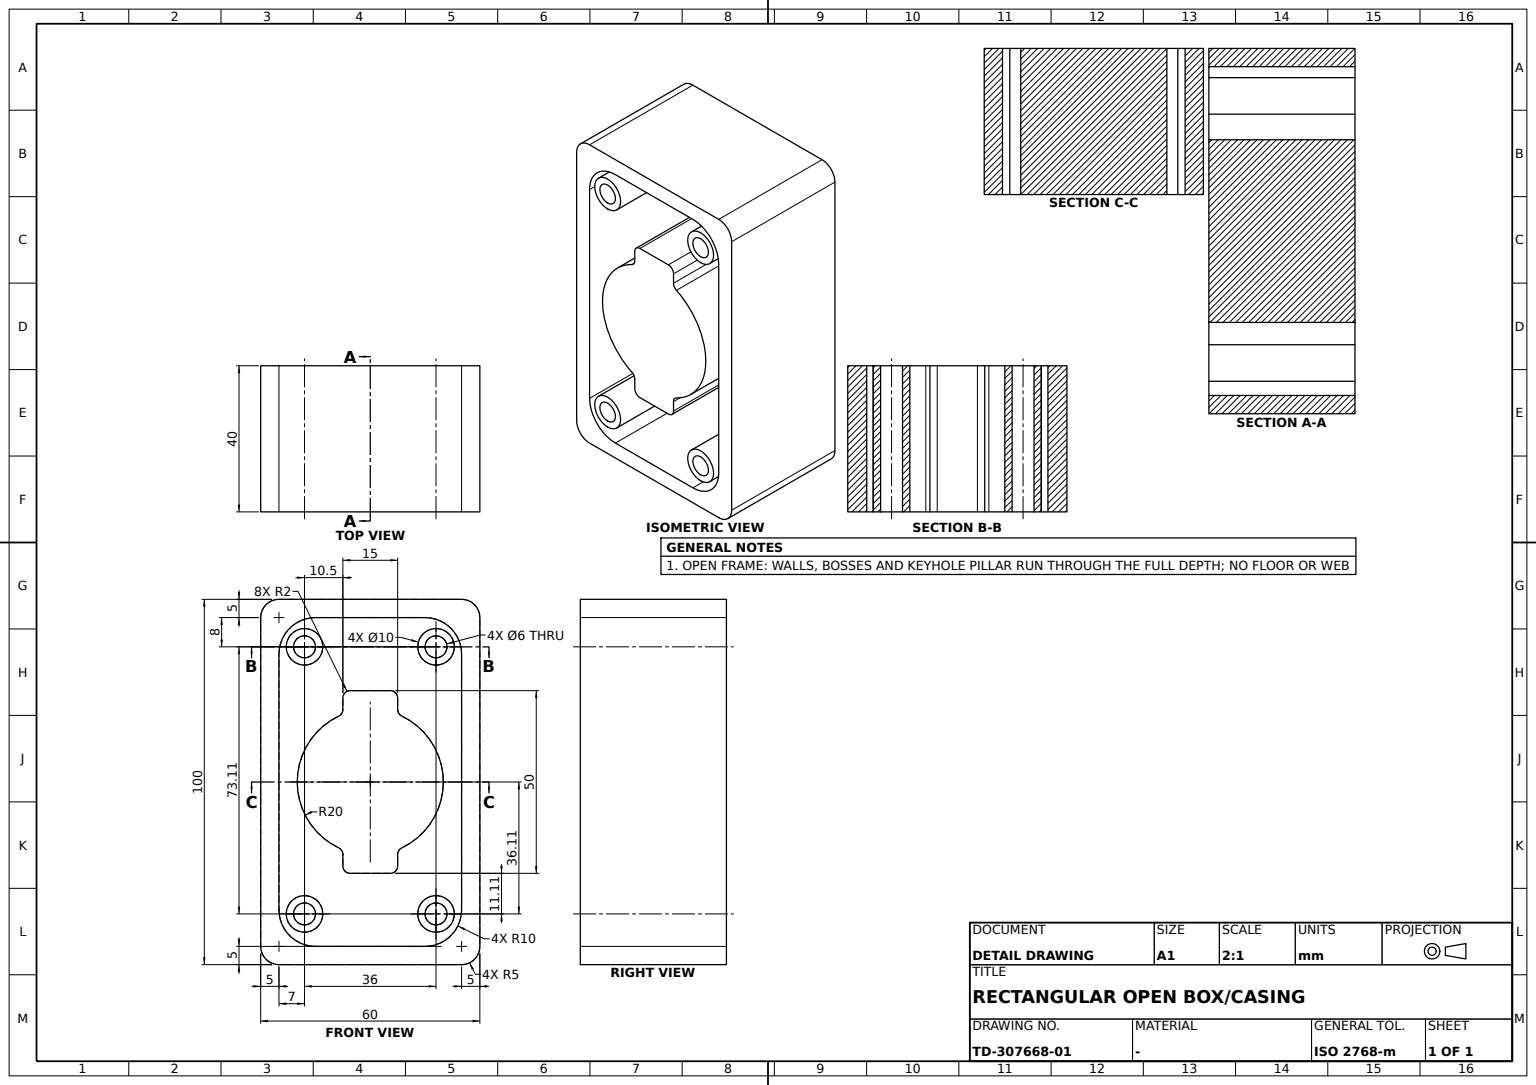
ISO-10303-21;
HEADER;
FILE_DESCRIPTION((''),'2;1');
FILE_NAME('','',(''),(''),'','','');
FILE_SCHEMA(('AUTOMOTIVE_DESIGN'));
ENDSEC;
DATA;
#1=APPLICATION_CONTEXT('');
#2=PRODUCT_CONTEXT('',#1,'mechanical');
#3=PRODUCT('','','',(#2));
#4=PRODUCT_DEFINITION_FORMATION('','',#3);
#5=PRODUCT_DEFINITION_CONTEXT('',#1,'design');
#6=PRODUCT_DEFINITION('','',#4,#5);
#7=PRODUCT_DEFINITION_SHAPE('','',#6);
#8=(LENGTH_UNIT()NAMED_UNIT(*)SI_UNIT(.MILLI.,.METRE.));
#9=(NAMED_UNIT(*)PLANE_ANGLE_UNIT()SI_UNIT($,.RADIAN.));
#10=(NAMED_UNIT(*)SI_UNIT($,.STERADIAN.)SOLID_ANGLE_UNIT());
#11=UNCERTAINTY_MEASURE_WITH_UNIT(LENGTH_MEASURE(0.005),#8,'distance_accuracy_value','');
#12=(GEOMETRIC_REPRESENTATION_CONTEXT(3)GLOBAL_UNCERTAINTY_ASSIGNED_CONTEXT((#11))GLOBAL_UNIT_ASSIGNED_CONTEXT((#8,#9,#10))REPRESENTATION_CONTEXT('',''));
#13=CARTESIAN_POINT('',(20.,-18.,-41.111401));
#14=VERTEX_POINT('',#13);
#15=CARTESIAN_POINT('',(20.,-18.,-36.111401));
#16=DIRECTION('',(1.,0.,0.));
#17=DIRECTION('',(0.,0.,-1.));
#18=AXIS2_PLACEMENT_3D('',#15,#16,#17);
#19=CIRCLE('',#18,5.);
#20=EDGE_CURVE('',#14,#14,#19,.T.);
#21=ORIENTED_EDGE('',*,*,#20,.T.);
#22=EDGE_LOOP('',(#21));
#23=FACE_BOUND('',#22,.T.);
#24=CARTESIAN_POINT('',(20.,-18.,-39.111401));
#25=VERTEX_POINT('',#24);
#26=CIRCLE('',#18,3.);
#27=EDGE_CURVE('',#25,#25,#26,.T.);
#28=ORIENTED_EDGE('',*,*,#27,.F.);
#29=EDGE_LOOP('',(#28));
#30=FACE_BOUND('',#29,.T.);
#31=CARTESIAN_POINT('',(20.,0.,0.));
#32=DIRECTION('',(0.,1.,0.));
#33=AXIS2_PLACEMENT_3D('',#31,#16,#32);
#34=PLANE('',#33);
#35=ADVANCED_FACE('',(#23,#30),#34,.T.);
#36=ORIENTED_EDGE('',*,*,#20,.F.);
#37=EDGE_LOOP('',(#36));
#38=FACE_BOUND('',#37,.T.);
#39=CARTESIAN_POINT('',(-20.,-18.,-41.111401));
#40=VERTEX_POINT('',#39);
#41=CARTESIAN_POINT('',(-20.,-18.,-36.111401));
#42=AXIS2_PLACEMENT_3D('',#41,#16,#17);
#43=CIRCLE('',#42,5.);
#44=EDGE_CURVE('',#40,#40,#43,.T.);
#45=ORIENTED_EDGE('',*,*,#44,.T.);
#46=EDGE_LOOP('',(#45));
#47=FACE_BOUND('',#46,.T.);
#48=CARTESIAN_POINT('',(0.,-18.,-36.111401));
#49=AXIS2_PLACEMENT_3D('',#48,#16,#32);
#50=CYLINDRICAL_SURFACE('',#49,5.);
#51=ADVANCED_FACE('',(#38,#47),#50,.T.);
#52=ORIENTED_EDGE('',*,*,#44,.F.);
#53=EDGE_LOOP('',(#52));
#54=FACE_BOUND('',#53,.T.);
#55=CARTESIAN_POINT('',(-20.,-18.,-39.111401));
#56=VERTEX_POINT('',#55);
#57=CIRCLE('',#42,3.);
#58=EDGE_CURVE('',#56,#56,#57,.T.);
#59=ORIENTED_EDGE('',*,*,#58,.T.);
#60=EDGE_LOOP('',(#59));
#61=FACE_BOUND('',#60,.T.);
#62=CARTESIAN_POINT('',(-20.,0.,0.));
#63=AXIS2_PLACEMENT_3D('',#62,#16,#32);
#64=PLANE('',#63);
#65=ADVANCED_FACE('',(#54,#61),#64,.F.);
#66=ORIENTED_EDGE('',*,*,#27,.T.);
#67=EDGE_LOOP('',(#66));
#68=FACE_BOUND('',#67,.T.);
#69=ORIENTED_EDGE('',*,*,#58,.F.);
#70=EDGE_LOOP('',(#69));
#71=FACE_BOUND('',#70,.T.);
#72=CYLINDRICAL_SURFACE('',#49,3.);
#73=ADVANCED_FACE('',(#68,#71),#72,.F.);
#74=CLOSED_SHELL('',(#35,#51,#65,#73));
#75=MANIFOLD_SOLID_BREP('',#74);
#76=CARTESIAN_POINT('',(-20.,30.,45.));
#77=VERTEX_POINT('',#76);
#78=CARTESIAN_POINT('',(20.,30.,45.));
#79=VERTEX_POINT('',#78);
#80=CARTESIAN_POINT('',(0.,30.,45.));
#81=VECTOR('',#16,1000.);
#82=LINE('',#80,#81);
#83=EDGE_CURVE('',#77,#79,#82,.T.);
#84=ORIENTED_EDGE('',*,*,#83,.T.);
#85=CARTESIAN_POINT('',(20.,30.,-45.));
#86=VERTEX_POINT('',#85);
#87=CARTESIAN_POINT('',(20.,30.,0.));
#88=DIRECTION('',(0.,0.,1.));
#89=VECTOR('',#88,1000.);
#90=LINE('',#87,#89);
#91=EDGE_CURVE('',#86,#79,#90,.T.);
#92=ORIENTED_EDGE('',*,*,#91,.F.);
#93=CARTESIAN_POINT('',(-20.,30.,-45.));
#94=VERTEX_POINT('',#93);
#95=CARTESIAN_POINT('',(0.,30.,-45.));
#96=LINE('',#95,#81);
#97=EDGE_CURVE('',#94,#86,#96,.T.);
#98=ORIENTED_EDGE('',*,*,#97,.F.);
#99=CARTESIAN_POINT('',(-20.,30.,0.));
#100=LINE('',#99,#89);
#101=EDGE_CURVE('',#94,#77,#100,.T.);
#102=ORIENTED_EDGE('',*,*,#101,.T.);
#103=EDGE_LOOP('',(#84,#92,#98,#102));
#104=FACE_BOUND('',#103,.T.);
#105=CARTESIAN_POINT('',(0.,30.,-50.));
#106=AXIS2_PLACEMENT_3D('',#105,#32,#88);
#107=PLANE('',#106);
#108=ADVANCED_FACE('',(#104),#107,.T.);
#109=CARTESIAN_POINT('',(-20.,25.,35.));
#110=VERTEX_POINT('',#109);
#111=CARTESIAN_POINT('',(20.,25.,35.));
#112=VERTEX_POINT('',#111);
#113=CARTESIAN_POINT('',(0.,25.,35.));
#114=LINE('',#113,#81);
#115=EDGE_CURVE('',#110,#112,#114,.T.);
#116=ORIENTED_EDGE('',*,*,#115,.F.);
#117=CARTESIAN_POINT('',(-20.,25.,-35.));
#118=VERTEX_POINT('',#117);
#119=CARTESIAN_POINT('',(-20.,25.,0.));
#120=LINE('',#119,#89);
#121=EDGE_CURVE('',#118,#110,#120,.T.);
#122=ORIENTED_EDGE('',*,*,#121,.F.);
#123=CARTESIAN_POINT('',(20.,25.,-35.));
#124=VERTEX_POINT('',#123);
#125=CARTESIAN_POINT('',(0.,25.,-35.));
#126=LINE('',#125,#81);
#127=EDGE_CURVE('',#118,#124,#126,.T.);
#128=ORIENTED_EDGE('',*,*,#127,.T.);
#129=CARTESIAN_POINT('',(20.,25.,0.));
#130=LINE('',#129,#89);
#131=EDGE_CURVE('',#124,#112,#130,.T.);
#132=ORIENTED_EDGE('',*,*,#131,.T.);
#133=EDGE_LOOP('',(#116,#122,#128,#132));
#134=FACE_BOUND('',#133,.T.);
#135=CARTESIAN_POINT('',(0.,25.,-45.));
#136=AXIS2_PLACEMENT_3D('',#135,#32,#88);
#137=PLANE('',#136);
#138=ADVANCED_FACE('',(#134),#137,.F.);
#139=CARTESIAN_POINT('',(-20.,-30.,-45.));
#140=VERTEX_POINT('',#139);
#141=CARTESIAN_POINT('',(20.,-30.,-45.));
#142=VERTEX_POINT('',#141);
#143=CARTESIAN_POINT('',(0.,-30.,-45.));
#144=LINE('',#143,#81);
#145=EDGE_CURVE('',#140,#142,#144,.T.);
#146=ORIENTED_EDGE('',*,*,#145,.F.);
#147=CARTESIAN_POINT('',(-20.,-25.,-50.));
#148=VERTEX_POINT('',#147);
#149=CARTESIAN_POINT('',(-20.,-25.,-45.));
#150=AXIS2_PLACEMENT_3D('',#149,#16,#17);
#151=CIRCLE('',#150,5.);
#152=EDGE_CURVE('',#140,#148,#151,.T.);
#153=ORIENTED_EDGE('',*,*,#152,.T.);
#154=CARTESIAN_POINT('',(20.,-25.,-50.));
#155=VERTEX_POINT('',#154);
#156=CARTESIAN_POINT('',(0.,-25.,-50.));
#157=LINE('',#156,#81);
#158=EDGE_CURVE('',#148,#155,#157,.T.);
#159=ORIENTED_EDGE('',*,*,#158,.T.);
#160=CARTESIAN_POINT('',(20.,-25.,-45.));
#161=AXIS2_PLACEMENT_3D('',#160,#16,#17);
#162=CIRCLE('',#161,5.);
#163=EDGE_CURVE('',#142,#155,#162,.T.);
#164=ORIENTED_EDGE('',*,*,#163,.F.);
#165=EDGE_LOOP('',(#146,#153,#159,#164));
#166=FACE_BOUND('',#165,.T.);
#167=CARTESIAN_POINT('',(0.,-25.,-45.));
#168=AXIS2_PLACEMENT_3D('',#167,#16,#17);
#169=CYLINDRICAL_SURFACE('',#168,5.);
#170=ADVANCED_FACE('',(#166),#169,.T.);
#171=CARTESIAN_POINT('',(20.,15.,-45.));
#172=VERTEX_POINT('',#171);
#173=CARTESIAN_POINT('',(20.,15.,-35.));
#174=AXIS2_PLACEMENT_3D('',#173,#16,#17);
#175=CIRCLE('',#174,10.);
#176=EDGE_CURVE('',#172,#124,#175,.T.);
#177=ORIENTED_EDGE('',*,*,#176,.T.);
#178=ORIENTED_EDGE('',*,*,#127,.F.);
#179=CARTESIAN_POINT('',(-20.,15.,-45.));
#180=VERTEX_POINT('',#179);
#181=CARTESIAN_POINT('',(-20.,15.,-35.));
#182=AXIS2_PLACEMENT_3D('',#181,#16,#17);
#183=CIRCLE('',#182,10.);
#184=EDGE_CURVE('',#180,#118,#183,.T.);
#185=ORIENTED_EDGE('',*,*,#184,.F.);
#186=CARTESIAN_POINT('',(0.,15.,-45.));
#187=LINE('',#186,#81);
#188=EDGE_CURVE('',#180,#172,#187,.T.);
#189=ORIENTED_EDGE('',*,*,#188,.T.);
#190=EDGE_LOOP('',(#177,#178,#185,#189));
#191=FACE_BOUND('',#190,.T.);
#192=CARTESIAN_POINT('',(0.,15.,-35.));
#193=AXIS2_PLACEMENT_3D('',#192,#16,#17);
#194=CYLINDRICAL_SURFACE('',#193,10.);
#195=ADVANCED_FACE('',(#191),#194,.F.);
#196=CARTESIAN_POINT('',(20.,25.,-50.));
#197=VERTEX_POINT('',#196);
#198=CARTESIAN_POINT('',(20.,0.,-50.));
#199=DIRECTION('',(0.,-1.,0.));
#200=VECTOR('',#199,1000.);
#201=LINE('',#198,#200);
#202=EDGE_CURVE('',#197,#155,#201,.T.);
#203=ORIENTED_EDGE('',*,*,#202,.F.);
#204=CARTESIAN_POINT('',(20.,25.,-45.));
#205=AXIS2_PLACEMENT_3D('',#204,#16,#17);
#206=CIRCLE('',#205,5.);
#207=EDGE_CURVE('',#197,#86,#206,.T.);
#208=ORIENTED_EDGE('',*,*,#207,.T.);
#209=ORIENTED_EDGE('',*,*,#91,.T.);
#210=CARTESIAN_POINT('',(20.,25.,50.));
#211=VERTEX_POINT('',#210);
#212=CARTESIAN_POINT('',(20.,25.,45.));
#213=AXIS2_PLACEMENT_3D('',#212,#16,#17);
#214=CIRCLE('',#213,5.);
#215=EDGE_CURVE('',#79,#211,#214,.T.);
#216=ORIENTED_EDGE('',*,*,#215,.T.);
#217=CARTESIAN_POINT('',(20.,-25.,50.));
#218=VERTEX_POINT('',#217);
#219=CARTESIAN_POINT('',(20.,0.,50.));
#220=VECTOR('',#32,1000.);
#221=LINE('',#219,#220);
#222=EDGE_CURVE('',#218,#211,#221,.T.);
#223=ORIENTED_EDGE('',*,*,#222,.F.);
#224=CARTESIAN_POINT('',(20.,-30.,45.));
#225=VERTEX_POINT('',#224);
#226=CARTESIAN_POINT('',(20.,-25.,45.));
#227=AXIS2_PLACEMENT_3D('',#226,#16,#17);
#228=CIRCLE('',#227,5.);
#229=EDGE_CURVE('',#218,#225,#228,.T.);
#230=ORIENTED_EDGE('',*,*,#229,.T.);
#231=CARTESIAN_POINT('',(20.,-30.,0.));
#232=VECTOR('',#17,1000.);
#233=LINE('',#231,#232);
#234=EDGE_CURVE('',#225,#142,#233,.T.);
#235=ORIENTED_EDGE('',*,*,#234,.T.);
#236=ORIENTED_EDGE('',*,*,#163,.T.);
#237=EDGE_LOOP('',(#203,#208,#209,#216,#223,#230,#235,#236));
#238=FACE_BOUND('',#237,.T.);
#239=CARTESIAN_POINT('',(20.,-15.,45.));
#240=VERTEX_POINT('',#239);
#241=CARTESIAN_POINT('',(20.,-25.,35.));
#242=VERTEX_POINT('',#241);
#243=CARTESIAN_POINT('',(20.,-15.,35.));
#244=AXIS2_PLACEMENT_3D('',#243,#16,#17);
#245=CIRCLE('',#244,10.);
#246=EDGE_CURVE('',#240,#242,#245,.T.);
#247=ORIENTED_EDGE('',*,*,#246,.F.);
#248=CARTESIAN_POINT('',(20.,15.,45.));
#249=VERTEX_POINT('',#248);
#250=CARTESIAN_POINT('',(20.,0.,45.));
#251=LINE('',#250,#220);
#252=EDGE_CURVE('',#240,#249,#251,.T.);
#253=ORIENTED_EDGE('',*,*,#252,.T.);
#254=CARTESIAN_POINT('',(20.,15.,35.));
#255=AXIS2_PLACEMENT_3D('',#254,#16,#17);
#256=CIRCLE('',#255,10.);
#257=EDGE_CURVE('',#112,#249,#256,.T.);
#258=ORIENTED_EDGE('',*,*,#257,.F.);
#259=ORIENTED_EDGE('',*,*,#131,.F.);
#260=ORIENTED_EDGE('',*,*,#176,.F.);
#261=CARTESIAN_POINT('',(20.,-15.,-45.));
#262=VERTEX_POINT('',#261);
#263=CARTESIAN_POINT('',(20.,0.,-45.));
#264=LINE('',#263,#200);
#265=EDGE_CURVE('',#172,#262,#264,.T.);
#266=ORIENTED_EDGE('',*,*,#265,.T.);
#267=CARTESIAN_POINT('',(20.,-25.,-35.));
#268=VERTEX_POINT('',#267);
#269=CARTESIAN_POINT('',(20.,-15.,-35.));
#270=AXIS2_PLACEMENT_3D('',#269,#16,#17);
#271=CIRCLE('',#270,10.);
#272=EDGE_CURVE('',#268,#262,#271,.T.);
#273=ORIENTED_EDGE('',*,*,#272,.F.);
#274=CARTESIAN_POINT('',(20.,-25.,0.));
#275=LINE('',#274,#232);
#276=EDGE_CURVE('',#242,#268,#275,.T.);
#277=ORIENTED_EDGE('',*,*,#276,.F.);
#278=EDGE_LOOP('',(#247,#253,#258,#259,#260,#266,#273,#277));
#279=FACE_BOUND('',#278,.T.);
#280=ADVANCED_FACE('',(#238,#279),#34,.T.);
#281=ORIENTED_EDGE('',*,*,#252,.F.);
#282=CARTESIAN_POINT('',(-20.,-15.,45.));
#283=VERTEX_POINT('',#282);
#284=CARTESIAN_POINT('',(0.,-15.,45.));
#285=LINE('',#284,#81);
#286=EDGE_CURVE('',#283,#240,#285,.T.);
#287=ORIENTED_EDGE('',*,*,#286,.F.);
#288=CARTESIAN_POINT('',(-20.,15.,45.));
#289=VERTEX_POINT('',#288);
#290=CARTESIAN_POINT('',(-20.,0.,45.));
#291=LINE('',#290,#220);
#292=EDGE_CURVE('',#283,#289,#291,.T.);
#293=ORIENTED_EDGE('',*,*,#292,.T.);
#294=CARTESIAN_POINT('',(0.,15.,45.));
#295=LINE('',#294,#81);
#296=EDGE_CURVE('',#289,#249,#295,.T.);
#297=ORIENTED_EDGE('',*,*,#296,.T.);
#298=EDGE_LOOP('',(#281,#287,#293,#297));
#299=FACE_BOUND('',#298,.T.);
#300=CARTESIAN_POINT('',(0.,-25.,45.));
#301=AXIS2_PLACEMENT_3D('',#300,#17,#32);
#302=PLANE('',#301);
#303=ADVANCED_FACE('',(#299),#302,.T.);
#304=CARTESIAN_POINT('',(-20.,-25.,50.));
#305=VERTEX_POINT('',#304);
#306=CARTESIAN_POINT('',(-20.,-30.,45.));
#307=VERTEX_POINT('',#306);
#308=CARTESIAN_POINT('',(-20.,-25.,45.));
#309=AXIS2_PLACEMENT_3D('',#308,#16,#17);
#310=CIRCLE('',#309,5.);
#311=EDGE_CURVE('',#305,#307,#310,.T.);
#312=ORIENTED_EDGE('',*,*,#311,.T.);
#313=CARTESIAN_POINT('',(0.,-30.,45.));
#314=LINE('',#313,#81);
#315=EDGE_CURVE('',#307,#225,#314,.T.);
#316=ORIENTED_EDGE('',*,*,#315,.T.);
#317=ORIENTED_EDGE('',*,*,#229,.F.);
#318=CARTESIAN_POINT('',(0.,-25.,50.));
#319=LINE('',#318,#81);
#320=EDGE_CURVE('',#305,#218,#319,.T.);
#321=ORIENTED_EDGE('',*,*,#320,.F.);
#322=EDGE_LOOP('',(#312,#316,#317,#321));
#323=FACE_BOUND('',#322,.T.);
#324=AXIS2_PLACEMENT_3D('',#300,#16,#199);
#325=CYLINDRICAL_SURFACE('',#324,5.);
#326=ADVANCED_FACE('',(#323),#325,.T.);
#327=CARTESIAN_POINT('',(-20.,-25.,35.));
#328=VERTEX_POINT('',#327);
#329=CARTESIAN_POINT('',(0.,-25.,35.));
#330=LINE('',#329,#81);
#331=EDGE_CURVE('',#328,#242,#330,.T.);
#332=ORIENTED_EDGE('',*,*,#331,.T.);
#333=ORIENTED_EDGE('',*,*,#276,.T.);
#334=CARTESIAN_POINT('',(-20.,-25.,-35.));
#335=VERTEX_POINT('',#334);
#336=CARTESIAN_POINT('',(0.,-25.,-35.));
#337=LINE('',#336,#81);
#338=EDGE_CURVE('',#335,#268,#337,.T.);
#339=ORIENTED_EDGE('',*,*,#338,.F.);
#340=CARTESIAN_POINT('',(-20.,-25.,0.));
#341=LINE('',#340,#232);
#342=EDGE_CURVE('',#328,#335,#341,.T.);
#343=ORIENTED_EDGE('',*,*,#342,.F.);
#344=EDGE_LOOP('',(#332,#333,#339,#343));
#345=FACE_BOUND('',#344,.T.);
#346=AXIS2_PLACEMENT_3D('',#300,#199,#17);
#347=PLANE('',#346);
#348=ADVANCED_FACE('',(#345),#347,.F.);
#349=CARTESIAN_POINT('',(-20.,-15.,-45.));
#350=VERTEX_POINT('',#349);
#351=CARTESIAN_POINT('',(0.,-15.,-45.));
#352=LINE('',#351,#81);
#353=EDGE_CURVE('',#350,#262,#352,.T.);
#354=ORIENTED_EDGE('',*,*,#353,.F.);
#355=CARTESIAN_POINT('',(-20.,-15.,-35.));
#356=AXIS2_PLACEMENT_3D('',#355,#16,#17);
#357=CIRCLE('',#356,10.);
#358=EDGE_CURVE('',#335,#350,#357,.T.);
#359=ORIENTED_EDGE('',*,*,#358,.F.);
#360=ORIENTED_EDGE('',*,*,#338,.T.);
#361=ORIENTED_EDGE('',*,*,#272,.T.);
#362=EDGE_LOOP('',(#354,#359,#360,#361));
#363=FACE_BOUND('',#362,.T.);
#364=CARTESIAN_POINT('',(0.,-15.,-35.));
#365=AXIS2_PLACEMENT_3D('',#364,#16,#199);
#366=CYLINDRICAL_SURFACE('',#365,10.);
#367=ADVANCED_FACE('',(#363),#366,.F.);
#368=ORIENTED_EDGE('',*,*,#234,.F.);
#369=ORIENTED_EDGE('',*,*,#315,.F.);
#370=CARTESIAN_POINT('',(-20.,-30.,0.));
#371=LINE('',#370,#232);
#372=EDGE_CURVE('',#307,#140,#371,.T.);
#373=ORIENTED_EDGE('',*,*,#372,.T.);
#374=ORIENTED_EDGE('',*,*,#145,.T.);
#375=EDGE_LOOP('',(#368,#369,#373,#374));
#376=FACE_BOUND('',#375,.T.);
#377=CARTESIAN_POINT('',(0.,-30.,50.));
#378=AXIS2_PLACEMENT_3D('',#377,#199,#17);
#379=PLANE('',#378);
#380=ADVANCED_FACE('',(#376),#379,.T.);
#381=ORIENTED_EDGE('',*,*,#331,.F.);
#382=CARTESIAN_POINT('',(-20.,-15.,35.));
#383=AXIS2_PLACEMENT_3D('',#382,#16,#17);
#384=CIRCLE('',#383,10.);
#385=EDGE_CURVE('',#283,#328,#384,.T.);
#386=ORIENTED_EDGE('',*,*,#385,.F.);
#387=ORIENTED_EDGE('',*,*,#286,.T.);
#388=ORIENTED_EDGE('',*,*,#246,.T.);
#389=EDGE_LOOP('',(#381,#386,#387,#388));
#390=FACE_BOUND('',#389,.T.);
#391=CARTESIAN_POINT('',(0.,-15.,35.));
#392=AXIS2_PLACEMENT_3D('',#391,#16,#88);
#393=CYLINDRICAL_SURFACE('',#392,10.);
#394=ADVANCED_FACE('',(#390),#393,.F.);
#395=ORIENTED_EDGE('',*,*,#353,.T.);
#396=ORIENTED_EDGE('',*,*,#265,.F.);
#397=ORIENTED_EDGE('',*,*,#188,.F.);
#398=CARTESIAN_POINT('',(-20.,0.,-45.));
#399=LINE('',#398,#200);
#400=EDGE_CURVE('',#180,#350,#399,.T.);
#401=ORIENTED_EDGE('',*,*,#400,.T.);
#402=EDGE_LOOP('',(#395,#396,#397,#401));
#403=FACE_BOUND('',#402,.T.);
#404=AXIS2_PLACEMENT_3D('',#135,#88,#199);
#405=PLANE('',#404);
#406=ADVANCED_FACE('',(#403),#405,.T.);
#407=CARTESIAN_POINT('',(-20.,25.,50.));
#408=VERTEX_POINT('',#407);
#409=CARTESIAN_POINT('',(0.,25.,50.));
#410=LINE('',#409,#81);
#411=EDGE_CURVE('',#408,#211,#410,.T.);
#412=ORIENTED_EDGE('',*,*,#411,.F.);
#413=CARTESIAN_POINT('',(-20.,0.,50.));
#414=LINE('',#413,#220);
#415=EDGE_CURVE('',#305,#408,#414,.T.);
#416=ORIENTED_EDGE('',*,*,#415,.F.);
#417=ORIENTED_EDGE('',*,*,#320,.T.);
#418=ORIENTED_EDGE('',*,*,#222,.T.);
#419=EDGE_LOOP('',(#412,#416,#417,#418));
#420=FACE_BOUND('',#419,.T.);
#421=AXIS2_PLACEMENT_3D('',#377,#17,#32);
#422=PLANE('',#421);
#423=ADVANCED_FACE('',(#420),#422,.F.);
#424=ORIENTED_EDGE('',*,*,#202,.T.);
#425=ORIENTED_EDGE('',*,*,#158,.F.);
#426=CARTESIAN_POINT('',(-20.,25.,-50.));
#427=VERTEX_POINT('',#426);
#428=CARTESIAN_POINT('',(-20.,0.,-50.));
#429=LINE('',#428,#200);
#430=EDGE_CURVE('',#427,#148,#429,.T.);
#431=ORIENTED_EDGE('',*,*,#430,.F.);
#432=CARTESIAN_POINT('',(0.,25.,-50.));
#433=LINE('',#432,#81);
#434=EDGE_CURVE('',#427,#197,#433,.T.);
#435=ORIENTED_EDGE('',*,*,#434,.T.);
#436=EDGE_LOOP('',(#424,#425,#431,#435));
#437=FACE_BOUND('',#436,.T.);
#438=AXIS2_PLACEMENT_3D('',#105,#88,#199);
#439=PLANE('',#438);
#440=ADVANCED_FACE('',(#437),#439,.F.);
#441=ORIENTED_EDGE('',*,*,#415,.T.);
#442=CARTESIAN_POINT('',(-20.,25.,45.));
#443=AXIS2_PLACEMENT_3D('',#442,#16,#17);
#444=CIRCLE('',#443,5.);
#445=EDGE_CURVE('',#77,#408,#444,.T.);
#446=ORIENTED_EDGE('',*,*,#445,.F.);
#447=ORIENTED_EDGE('',*,*,#101,.F.);
#448=CARTESIAN_POINT('',(-20.,25.,-45.));
#449=AXIS2_PLACEMENT_3D('',#448,#16,#17);
#450=CIRCLE('',#449,5.);
#451=EDGE_CURVE('',#427,#94,#450,.T.);
#452=ORIENTED_EDGE('',*,*,#451,.F.);
#453=ORIENTED_EDGE('',*,*,#430,.T.);
#454=ORIENTED_EDGE('',*,*,#152,.F.);
#455=ORIENTED_EDGE('',*,*,#372,.F.);
#456=ORIENTED_EDGE('',*,*,#311,.F.);
#457=EDGE_LOOP('',(#441,#446,#447,#452,#453,#454,#455,#456));
#458=FACE_BOUND('',#457,.T.);
#459=ORIENTED_EDGE('',*,*,#342,.T.);
#460=ORIENTED_EDGE('',*,*,#358,.T.);
#461=ORIENTED_EDGE('',*,*,#400,.F.);
#462=ORIENTED_EDGE('',*,*,#184,.T.);
#463=ORIENTED_EDGE('',*,*,#121,.T.);
#464=CARTESIAN_POINT('',(-20.,15.,35.));
#465=AXIS2_PLACEMENT_3D('',#464,#16,#17);
#466=CIRCLE('',#465,10.);
#467=EDGE_CURVE('',#110,#289,#466,.T.);
#468=ORIENTED_EDGE('',*,*,#467,.T.);
#469=ORIENTED_EDGE('',*,*,#292,.F.);
#470=ORIENTED_EDGE('',*,*,#385,.T.);
#471=EDGE_LOOP('',(#459,#460,#461,#462,#463,#468,#469,#470));
#472=FACE_BOUND('',#471,.T.);
#473=ADVANCED_FACE('',(#458,#472),#64,.F.);
#474=ORIENTED_EDGE('',*,*,#411,.T.);
#475=ORIENTED_EDGE('',*,*,#215,.F.);
#476=ORIENTED_EDGE('',*,*,#83,.F.);
#477=ORIENTED_EDGE('',*,*,#445,.T.);
#478=EDGE_LOOP('',(#474,#475,#476,#477));
#479=FACE_BOUND('',#478,.T.);
#480=CARTESIAN_POINT('',(0.,25.,45.));
#481=AXIS2_PLACEMENT_3D('',#480,#16,#88);
#482=CYLINDRICAL_SURFACE('',#481,5.);
#483=ADVANCED_FACE('',(#479),#482,.T.);
#484=ORIENTED_EDGE('',*,*,#451,.T.);
#485=ORIENTED_EDGE('',*,*,#97,.T.);
#486=ORIENTED_EDGE('',*,*,#207,.F.);
#487=ORIENTED_EDGE('',*,*,#434,.F.);
#488=EDGE_LOOP('',(#484,#485,#486,#487));
#489=FACE_BOUND('',#488,.T.);
#490=AXIS2_PLACEMENT_3D('',#135,#16,#32);
#491=CYLINDRICAL_SURFACE('',#490,5.);
#492=ADVANCED_FACE('',(#489),#491,.T.);
#493=ORIENTED_EDGE('',*,*,#296,.F.);
#494=ORIENTED_EDGE('',*,*,#467,.F.);
#495=ORIENTED_EDGE('',*,*,#115,.T.);
#496=ORIENTED_EDGE('',*,*,#257,.T.);
#497=EDGE_LOOP('',(#493,#494,#495,#496));
#498=FACE_BOUND('',#497,.T.);
#499=CARTESIAN_POINT('',(0.,15.,35.));
#500=AXIS2_PLACEMENT_3D('',#499,#16,#32);
#501=CYLINDRICAL_SURFACE('',#500,10.);
#502=ADVANCED_FACE('',(#498),#501,.F.);
#503=CLOSED_SHELL('',(#108,#138,#170,#195,#280,#303,#326,#348,#367,#380,#394,#406,#423,#440,#473,#483,#492,#502));
#504=MANIFOLD_SOLID_BREP('',#503);
#505=CARTESIAN_POINT('',(-20.,-18.,34.));
#506=VERTEX_POINT('',#505);
#507=CARTESIAN_POINT('',(-20.,-18.,37.));
#508=AXIS2_PLACEMENT_3D('',#507,#16,#17);
#509=CIRCLE('',#508,3.);
#510=EDGE_CURVE('',#506,#506,#509,.T.);
#511=ORIENTED_EDGE('',*,*,#510,.T.);
#512=EDGE_LOOP('',(#511));
#513=FACE_BOUND('',#512,.T.);
#514=CARTESIAN_POINT('',(-20.,-18.,32.));
#515=VERTEX_POINT('',#514);
#516=CIRCLE('',#508,5.);
#517=EDGE_CURVE('',#515,#515,#516,.T.);
#518=ORIENTED_EDGE('',*,*,#517,.F.);
#519=EDGE_LOOP('',(#518));
#520=FACE_BOUND('',#519,.T.);
#521=ADVANCED_FACE('',(#513,#520),#64,.F.);
#522=ORIENTED_EDGE('',*,*,#510,.F.);
#523=EDGE_LOOP('',(#522));
#524=FACE_BOUND('',#523,.T.);
#525=CARTESIAN_POINT('',(20.,-18.,34.));
#526=VERTEX_POINT('',#525);
#527=CARTESIAN_POINT('',(20.,-18.,37.));
#528=AXIS2_PLACEMENT_3D('',#527,#16,#17);
#529=CIRCLE('',#528,3.);
#530=EDGE_CURVE('',#526,#526,#529,.T.);
#531=ORIENTED_EDGE('',*,*,#530,.T.);
#532=EDGE_LOOP('',(#531));
#533=FACE_BOUND('',#532,.T.);
#534=CARTESIAN_POINT('',(0.,-18.,37.));
#535=AXIS2_PLACEMENT_3D('',#534,#16,#32);
#536=CYLINDRICAL_SURFACE('',#535,3.);
#537=ADVANCED_FACE('',(#524,#533),#536,.F.);
#538=CARTESIAN_POINT('',(20.,-18.,32.));
#539=VERTEX_POINT('',#538);
#540=CIRCLE('',#528,5.);
#541=EDGE_CURVE('',#539,#539,#540,.T.);
#542=ORIENTED_EDGE('',*,*,#541,.T.);
#543=EDGE_LOOP('',(#542));
#544=FACE_BOUND('',#543,.T.);
#545=ORIENTED_EDGE('',*,*,#530,.F.);
#546=EDGE_LOOP('',(#545));
#547=FACE_BOUND('',#546,.T.);
#548=ADVANCED_FACE('',(#544,#547),#34,.T.);
#549=ORIENTED_EDGE('',*,*,#541,.F.);
#550=EDGE_LOOP('',(#549));
#551=FACE_BOUND('',#550,.T.);
#552=ORIENTED_EDGE('',*,*,#517,.T.);
#553=EDGE_LOOP('',(#552));
#554=FACE_BOUND('',#553,.T.);
#555=CYLINDRICAL_SURFACE('',#535,5.);
#556=ADVANCED_FACE('',(#551,#554),#555,.T.);
#557=CLOSED_SHELL('',(#521,#537,#548,#556));
#558=MANIFOLD_SOLID_BREP('',#557);
#559=CARTESIAN_POINT('',(-20.,18.,-41.111401));
#560=VERTEX_POINT('',#559);
#561=CARTESIAN_POINT('',(-20.,18.,-36.111401));
#562=AXIS2_PLACEMENT_3D('',#561,#16,#17);
#563=CIRCLE('',#562,5.);
#564=EDGE_CURVE('',#560,#560,#563,.T.);
#565=ORIENTED_EDGE('',*,*,#564,.T.);
#566=EDGE_LOOP('',(#565));
#567=FACE_BOUND('',#566,.T.);
#568=CARTESIAN_POINT('',(20.,18.,-41.111401));
#569=VERTEX_POINT('',#568);
#570=CARTESIAN_POINT('',(20.,18.,-36.111401));
#571=AXIS2_PLACEMENT_3D('',#570,#16,#17);
#572=CIRCLE('',#571,5.);
#573=EDGE_CURVE('',#569,#569,#572,.T.);
#574=ORIENTED_EDGE('',*,*,#573,.F.);
#575=EDGE_LOOP('',(#574));
#576=FACE_BOUND('',#575,.T.);
#577=CARTESIAN_POINT('',(0.,18.,-36.111401));
#578=AXIS2_PLACEMENT_3D('',#577,#16,#32);
#579=CYLINDRICAL_SURFACE('',#578,5.);
#580=ADVANCED_FACE('',(#567,#576),#579,.T.);
#581=CARTESIAN_POINT('',(20.,18.,-39.111401));
#582=VERTEX_POINT('',#581);
#583=CIRCLE('',#571,3.);
#584=EDGE_CURVE('',#582,#582,#583,.T.);
#585=ORIENTED_EDGE('',*,*,#584,.F.);
#586=EDGE_LOOP('',(#585));
#587=FACE_BOUND('',#586,.T.);
#588=ORIENTED_EDGE('',*,*,#573,.T.);
#589=EDGE_LOOP('',(#588));
#590=FACE_BOUND('',#589,.T.);
#591=ADVANCED_FACE('',(#587,#590),#34,.T.);
#592=ORIENTED_EDGE('',*,*,#584,.T.);
#593=EDGE_LOOP('',(#592));
#594=FACE_BOUND('',#593,.T.);
#595=CARTESIAN_POINT('',(-20.,18.,-39.111401));
#596=VERTEX_POINT('',#595);
#597=CIRCLE('',#562,3.);
#598=EDGE_CURVE('',#596,#596,#597,.T.);
#599=ORIENTED_EDGE('',*,*,#598,.F.);
#600=EDGE_LOOP('',(#599));
#601=FACE_BOUND('',#600,.T.);
#602=CYLINDRICAL_SURFACE('',#578,3.);
#603=ADVANCED_FACE('',(#594,#601),#602,.F.);
#604=ORIENTED_EDGE('',*,*,#598,.T.);
#605=EDGE_LOOP('',(#604));
#606=FACE_BOUND('',#605,.T.);
#607=ORIENTED_EDGE('',*,*,#564,.F.);
#608=EDGE_LOOP('',(#607));
#609=FACE_BOUND('',#608,.T.);
#610=ADVANCED_FACE('',(#606,#609),#64,.F.);
#611=CLOSED_SHELL('',(#580,#591,#603,#610));
#612=MANIFOLD_SOLID_BREP('',#611);
#613=CARTESIAN_POINT('',(20.,7.5,19.843135));
#614=VERTEX_POINT('',#613);
#615=CARTESIAN_POINT('',(20.,7.5,23.));
#616=VERTEX_POINT('',#615);
#617=CARTESIAN_POINT('',(20.,7.5,0.));
#618=LINE('',#617,#89);
#619=EDGE_CURVE('',#614,#616,#618,.T.);
#620=ORIENTED_EDGE('',*,*,#619,.T.);
#621=CARTESIAN_POINT('',(20.,5.5,25.));
#622=VERTEX_POINT('',#621);
#623=CARTESIAN_POINT('',(20.,5.5,23.));
#624=AXIS2_PLACEMENT_3D('',#623,#16,#17);
#625=CIRCLE('',#624,2.);
#626=EDGE_CURVE('',#616,#622,#625,.T.);
#627=ORIENTED_EDGE('',*,*,#626,.T.);
#628=CARTESIAN_POINT('',(20.,-5.5,25.));
#629=VERTEX_POINT('',#628);
#630=CARTESIAN_POINT('',(20.,0.,25.));
#631=LINE('',#630,#220);
#632=EDGE_CURVE('',#629,#622,#631,.T.);
#633=ORIENTED_EDGE('',*,*,#632,.F.);
#634=CARTESIAN_POINT('',(20.,-7.5,23.));
#635=VERTEX_POINT('',#634);
#636=CARTESIAN_POINT('',(20.,-5.5,23.));
#637=AXIS2_PLACEMENT_3D('',#636,#16,#17);
#638=CIRCLE('',#637,2.);
#639=EDGE_CURVE('',#629,#635,#638,.T.);
#640=ORIENTED_EDGE('',*,*,#639,.T.);
#641=CARTESIAN_POINT('',(20.,-7.5,19.843135));
#642=VERTEX_POINT('',#641);
#643=CARTESIAN_POINT('',(20.,-7.5,0.));
#644=LINE('',#643,#232);
#645=EDGE_CURVE('',#635,#642,#644,.T.);
#646=ORIENTED_EDGE('',*,*,#645,.T.);
#647=CARTESIAN_POINT('',(20.,-8.636364,18.039213));
#648=VERTEX_POINT('',#647);
#649=CARTESIAN_POINT('',(20.,-9.5,19.843135));
#650=AXIS2_PLACEMENT_3D('',#649,#16,#17);
#651=CIRCLE('',#650,2.);
#652=EDGE_CURVE('',#648,#642,#651,.T.);
#653=ORIENTED_EDGE('',*,*,#652,.F.);
#654=CARTESIAN_POINT('',(20.,-8.636364,-18.039213));
#655=VERTEX_POINT('',#654);
#656=AXIS2_PLACEMENT_3D('',#31,#16,#17);
#657=CIRCLE('',#656,20.);
#658=EDGE_CURVE('',#648,#655,#657,.T.);
#659=ORIENTED_EDGE('',*,*,#658,.T.);
#660=CARTESIAN_POINT('',(20.,-7.5,-19.843135));
#661=VERTEX_POINT('',#660);
#662=CARTESIAN_POINT('',(20.,-9.5,-19.843135));
#663=AXIS2_PLACEMENT_3D('',#662,#16,#17);
#664=CIRCLE('',#663,2.);
#665=EDGE_CURVE('',#661,#655,#664,.T.);
#666=ORIENTED_EDGE('',*,*,#665,.F.);
#667=CARTESIAN_POINT('',(20.,-7.5,-23.));
#668=VERTEX_POINT('',#667);
#669=EDGE_CURVE('',#661,#668,#644,.T.);
#670=ORIENTED_EDGE('',*,*,#669,.T.);
#671=CARTESIAN_POINT('',(20.,-5.5,-25.));
#672=VERTEX_POINT('',#671);
#673=CARTESIAN_POINT('',(20.,-5.5,-23.));
#674=AXIS2_PLACEMENT_3D('',#673,#16,#17);
#675=CIRCLE('',#674,2.);
#676=EDGE_CURVE('',#668,#672,#675,.T.);
#677=ORIENTED_EDGE('',*,*,#676,.T.);
#678=CARTESIAN_POINT('',(20.,5.5,-25.));
#679=VERTEX_POINT('',#678);
#680=CARTESIAN_POINT('',(20.,0.,-25.));
#681=LINE('',#680,#200);
#682=EDGE_CURVE('',#679,#672,#681,.T.);
#683=ORIENTED_EDGE('',*,*,#682,.F.);
#684=CARTESIAN_POINT('',(20.,7.5,-23.));
#685=VERTEX_POINT('',#684);
#686=CARTESIAN_POINT('',(20.,5.5,-23.));
#687=AXIS2_PLACEMENT_3D('',#686,#16,#17);
#688=CIRCLE('',#687,2.);
#689=EDGE_CURVE('',#679,#685,#688,.T.);
#690=ORIENTED_EDGE('',*,*,#689,.T.);
#691=CARTESIAN_POINT('',(20.,7.5,-19.843135));
#692=VERTEX_POINT('',#691);
#693=EDGE_CURVE('',#685,#692,#618,.T.);
#694=ORIENTED_EDGE('',*,*,#693,.T.);
#695=CARTESIAN_POINT('',(20.,8.636364,-18.039213));
#696=VERTEX_POINT('',#695);
#697=CARTESIAN_POINT('',(20.,9.5,-19.843135));
#698=AXIS2_PLACEMENT_3D('',#697,#16,#17);
#699=CIRCLE('',#698,2.);
#700=EDGE_CURVE('',#696,#692,#699,.T.);
#701=ORIENTED_EDGE('',*,*,#700,.F.);
#702=CARTESIAN_POINT('',(20.,8.636364,18.039213));
#703=VERTEX_POINT('',#702);
#704=EDGE_CURVE('',#696,#703,#657,.T.);
#705=ORIENTED_EDGE('',*,*,#704,.T.);
#706=CARTESIAN_POINT('',(20.,9.5,19.843135));
#707=AXIS2_PLACEMENT_3D('',#706,#16,#17);
#708=CIRCLE('',#707,2.);
#709=EDGE_CURVE('',#614,#703,#708,.T.);
#710=ORIENTED_EDGE('',*,*,#709,.F.);
#711=EDGE_LOOP('',(#620,#627,#633,#640,#646,#653,#659,#666,#670,#677,#683,#690,#694,#701,#705,#710));
#712=FACE_BOUND('',#711,.T.);
#713=ADVANCED_FACE('',(#712),#34,.T.);
#714=ORIENTED_EDGE('',*,*,#639,.F.);
#715=CARTESIAN_POINT('',(-20.,-5.5,25.));
#716=VERTEX_POINT('',#715);
#717=CARTESIAN_POINT('',(0.,-5.5,25.));
#718=LINE('',#717,#81);
#719=EDGE_CURVE('',#716,#629,#718,.T.);
#720=ORIENTED_EDGE('',*,*,#719,.F.);
#721=CARTESIAN_POINT('',(-20.,-7.5,23.));
#722=VERTEX_POINT('',#721);
#723=CARTESIAN_POINT('',(-20.,-5.5,23.));
#724=AXIS2_PLACEMENT_3D('',#723,#16,#17);
#725=CIRCLE('',#724,2.);
#726=EDGE_CURVE('',#716,#722,#725,.T.);
#727=ORIENTED_EDGE('',*,*,#726,.T.);
#728=CARTESIAN_POINT('',(0.,-7.5,23.));
#729=LINE('',#728,#81);
#730=EDGE_CURVE('',#722,#635,#729,.T.);
#731=ORIENTED_EDGE('',*,*,#730,.T.);
#732=EDGE_LOOP('',(#714,#720,#727,#731));
#733=FACE_BOUND('',#732,.T.);
#734=CARTESIAN_POINT('',(0.,-5.5,23.));
#735=AXIS2_PLACEMENT_3D('',#734,#16,#199);
#736=CYLINDRICAL_SURFACE('',#735,2.);
#737=ADVANCED_FACE('',(#733),#736,.T.);
#738=ORIENTED_EDGE('',*,*,#652,.T.);
#739=CARTESIAN_POINT('',(-20.,-7.5,19.843135));
#740=VERTEX_POINT('',#739);
#741=CARTESIAN_POINT('',(0.,-7.5,19.843135));
#742=LINE('',#741,#81);
#743=EDGE_CURVE('',#740,#642,#742,.T.);
#744=ORIENTED_EDGE('',*,*,#743,.F.);
#745=CARTESIAN_POINT('',(-20.,-8.636364,18.039213));
#746=VERTEX_POINT('',#745);
#747=CARTESIAN_POINT('',(-20.,-9.5,19.843135));
#748=AXIS2_PLACEMENT_3D('',#747,#16,#17);
#749=CIRCLE('',#748,2.);
#750=EDGE_CURVE('',#746,#740,#749,.T.);
#751=ORIENTED_EDGE('',*,*,#750,.F.);
#752=CARTESIAN_POINT('',(0.,-8.636364,18.039213));
#753=LINE('',#752,#81);
#754=EDGE_CURVE('',#746,#648,#753,.T.);
#755=ORIENTED_EDGE('',*,*,#754,.T.);
#756=EDGE_LOOP('',(#738,#744,#751,#755));
#757=FACE_BOUND('',#756,.T.);
#758=CARTESIAN_POINT('',(0.,-9.5,19.843135));
#759=DIRECTION('',(0.,0.431818182,-0.901960674));
#760=AXIS2_PLACEMENT_3D('',#758,#16,#759);
#761=CYLINDRICAL_SURFACE('',#760,2.);
#762=ADVANCED_FACE('',(#757),#761,.F.);
#763=CARTESIAN_POINT('',(-20.,8.636364,-18.039213));
#764=VERTEX_POINT('',#763);
#765=CARTESIAN_POINT('',(-20.,8.636364,18.039213));
#766=VERTEX_POINT('',#765);
#767=AXIS2_PLACEMENT_3D('',#62,#16,#17);
#768=CIRCLE('',#767,20.);
#769=EDGE_CURVE('',#764,#766,#768,.T.);
#770=ORIENTED_EDGE('',*,*,#769,.T.);
#771=CARTESIAN_POINT('',(0.,8.636364,18.039213));
#772=LINE('',#771,#81);
#773=EDGE_CURVE('',#766,#703,#772,.T.);
#774=ORIENTED_EDGE('',*,*,#773,.T.);
#775=ORIENTED_EDGE('',*,*,#704,.F.);
#776=CARTESIAN_POINT('',(0.,8.636364,-18.039213));
#777=LINE('',#776,#81);
#778=EDGE_CURVE('',#764,#696,#777,.T.);
#779=ORIENTED_EDGE('',*,*,#778,.F.);
#780=EDGE_LOOP('',(#770,#774,#775,#779));
#781=FACE_BOUND('',#780,.T.);
#782=CARTESIAN_POINT('',(0.,0.,0.));
#783=AXIS2_PLACEMENT_3D('',#782,#16,#32);
#784=CYLINDRICAL_SURFACE('',#783,20.);
#785=ADVANCED_FACE('',(#781),#784,.T.);
#786=CARTESIAN_POINT('',(-20.,7.5,19.843135));
#787=VERTEX_POINT('',#786);
#788=CARTESIAN_POINT('',(-20.,7.5,23.));
#789=VERTEX_POINT('',#788);
#790=CARTESIAN_POINT('',(-20.,7.5,0.));
#791=LINE('',#790,#89);
#792=EDGE_CURVE('',#787,#789,#791,.T.);
#793=ORIENTED_EDGE('',*,*,#792,.T.);
#794=CARTESIAN_POINT('',(0.,7.5,23.));
#795=LINE('',#794,#81);
#796=EDGE_CURVE('',#789,#616,#795,.T.);
#797=ORIENTED_EDGE('',*,*,#796,.T.);
#798=ORIENTED_EDGE('',*,*,#619,.F.);
#799=CARTESIAN_POINT('',(0.,7.5,19.843135));
#800=LINE('',#799,#81);
#801=EDGE_CURVE('',#787,#614,#800,.T.);
#802=ORIENTED_EDGE('',*,*,#801,.F.);
#803=EDGE_LOOP('',(#793,#797,#798,#802));
#804=FACE_BOUND('',#803,.T.);
#805=CARTESIAN_POINT('',(0.,7.5,-25.));
#806=AXIS2_PLACEMENT_3D('',#805,#32,#88);
#807=PLANE('',#806);
#808=ADVANCED_FACE('',(#804),#807,.T.);
#809=ORIENTED_EDGE('',*,*,#682,.T.);
#810=CARTESIAN_POINT('',(-20.,-5.5,-25.));
#811=VERTEX_POINT('',#810);
#812=CARTESIAN_POINT('',(0.,-5.5,-25.));
#813=LINE('',#812,#81);
#814=EDGE_CURVE('',#811,#672,#813,.T.);
#815=ORIENTED_EDGE('',*,*,#814,.F.);
#816=CARTESIAN_POINT('',(-20.,5.5,-25.));
#817=VERTEX_POINT('',#816);
#818=CARTESIAN_POINT('',(-20.,0.,-25.));
#819=LINE('',#818,#200);
#820=EDGE_CURVE('',#817,#811,#819,.T.);
#821=ORIENTED_EDGE('',*,*,#820,.F.);
#822=CARTESIAN_POINT('',(0.,5.5,-25.));
#823=LINE('',#822,#81);
#824=EDGE_CURVE('',#817,#679,#823,.T.);
#825=ORIENTED_EDGE('',*,*,#824,.T.);
#826=EDGE_LOOP('',(#809,#815,#821,#825));
#827=FACE_BOUND('',#826,.T.);
#828=AXIS2_PLACEMENT_3D('',#805,#88,#199);
#829=PLANE('',#828);
#830=ADVANCED_FACE('',(#827),#829,.F.);
#831=ORIENTED_EDGE('',*,*,#796,.F.);
#832=CARTESIAN_POINT('',(-20.,5.5,25.));
#833=VERTEX_POINT('',#832);
#834=CARTESIAN_POINT('',(-20.,5.5,23.));
#835=AXIS2_PLACEMENT_3D('',#834,#16,#17);
#836=CIRCLE('',#835,2.);
#837=EDGE_CURVE('',#789,#833,#836,.T.);
#838=ORIENTED_EDGE('',*,*,#837,.T.);
#839=CARTESIAN_POINT('',(0.,5.5,25.));
#840=LINE('',#839,#81);
#841=EDGE_CURVE('',#833,#622,#840,.T.);
#842=ORIENTED_EDGE('',*,*,#841,.T.);
#843=ORIENTED_EDGE('',*,*,#626,.F.);
#844=EDGE_LOOP('',(#831,#838,#842,#843));
#845=FACE_BOUND('',#844,.T.);
#846=CARTESIAN_POINT('',(0.,5.5,23.));
#847=AXIS2_PLACEMENT_3D('',#846,#16,#88);
#848=CYLINDRICAL_SURFACE('',#847,2.);
#849=ADVANCED_FACE('',(#845),#848,.T.);
#850=ORIENTED_EDGE('',*,*,#841,.F.);
#851=CARTESIAN_POINT('',(-20.,0.,25.));
#852=LINE('',#851,#220);
#853=EDGE_CURVE('',#716,#833,#852,.T.);
#854=ORIENTED_EDGE('',*,*,#853,.F.);
#855=ORIENTED_EDGE('',*,*,#719,.T.);
#856=ORIENTED_EDGE('',*,*,#632,.T.);
#857=EDGE_LOOP('',(#850,#854,#855,#856));
#858=FACE_BOUND('',#857,.T.);
#859=CARTESIAN_POINT('',(0.,-7.5,25.));
#860=AXIS2_PLACEMENT_3D('',#859,#17,#32);
#861=PLANE('',#860);
#862=ADVANCED_FACE('',(#858),#861,.F.);
#863=CARTESIAN_POINT('',(-20.,-7.5,-23.));
#864=VERTEX_POINT('',#863);
#865=CARTESIAN_POINT('',(0.,-7.5,-23.));
#866=LINE('',#865,#81);
#867=EDGE_CURVE('',#864,#668,#866,.T.);
#868=ORIENTED_EDGE('',*,*,#867,.F.);
#869=CARTESIAN_POINT('',(-20.,-5.5,-23.));
#870=AXIS2_PLACEMENT_3D('',#869,#16,#17);
#871=CIRCLE('',#870,2.);
#872=EDGE_CURVE('',#864,#811,#871,.T.);
#873=ORIENTED_EDGE('',*,*,#872,.T.);
#874=ORIENTED_EDGE('',*,*,#814,.T.);
#875=ORIENTED_EDGE('',*,*,#676,.F.);
#876=EDGE_LOOP('',(#868,#873,#874,#875));
#877=FACE_BOUND('',#876,.T.);
#878=CARTESIAN_POINT('',(0.,-5.5,-23.));
#879=AXIS2_PLACEMENT_3D('',#878,#16,#17);
#880=CYLINDRICAL_SURFACE('',#879,2.);
#881=ADVANCED_FACE('',(#877),#880,.T.);
#882=CARTESIAN_POINT('',(-20.,7.5,-23.));
#883=VERTEX_POINT('',#882);
#884=CARTESIAN_POINT('',(0.,7.5,-23.));
#885=LINE('',#884,#81);
#886=EDGE_CURVE('',#883,#685,#885,.T.);
#887=ORIENTED_EDGE('',*,*,#886,.T.);
#888=ORIENTED_EDGE('',*,*,#689,.F.);
#889=ORIENTED_EDGE('',*,*,#824,.F.);
#890=CARTESIAN_POINT('',(-20.,5.5,-23.));
#891=AXIS2_PLACEMENT_3D('',#890,#16,#17);
#892=CIRCLE('',#891,2.);
#893=EDGE_CURVE('',#817,#883,#892,.T.);
#894=ORIENTED_EDGE('',*,*,#893,.T.);
#895=EDGE_LOOP('',(#887,#888,#889,#894));
#896=FACE_BOUND('',#895,.T.);
#897=CARTESIAN_POINT('',(0.,5.5,-23.));
#898=AXIS2_PLACEMENT_3D('',#897,#16,#32);
#899=CYLINDRICAL_SURFACE('',#898,2.);
#900=ADVANCED_FACE('',(#896),#899,.T.);
#901=ORIENTED_EDGE('',*,*,#743,.T.);
#902=ORIENTED_EDGE('',*,*,#645,.F.);
#903=ORIENTED_EDGE('',*,*,#730,.F.);
#904=CARTESIAN_POINT('',(-20.,-7.5,0.));
#905=LINE('',#904,#232);
#906=EDGE_CURVE('',#722,#740,#905,.T.);
#907=ORIENTED_EDGE('',*,*,#906,.T.);
#908=EDGE_LOOP('',(#901,#902,#903,#907));
#909=FACE_BOUND('',#908,.T.);
#910=AXIS2_PLACEMENT_3D('',#859,#199,#17);
#911=PLANE('',#910);
#912=ADVANCED_FACE('',(#909),#911,.T.);
#913=ORIENTED_EDGE('',*,*,#778,.T.);
#914=ORIENTED_EDGE('',*,*,#700,.T.);
#915=CARTESIAN_POINT('',(-20.,7.5,-19.843135));
#916=VERTEX_POINT('',#915);
#917=CARTESIAN_POINT('',(0.,7.5,-19.843135));
#918=LINE('',#917,#81);
#919=EDGE_CURVE('',#916,#692,#918,.T.);
#920=ORIENTED_EDGE('',*,*,#919,.F.);
#921=CARTESIAN_POINT('',(-20.,9.5,-19.843135));
#922=AXIS2_PLACEMENT_3D('',#921,#16,#17);
#923=CIRCLE('',#922,2.);
#924=EDGE_CURVE('',#764,#916,#923,.T.);
#925=ORIENTED_EDGE('',*,*,#924,.F.);
#926=EDGE_LOOP('',(#913,#914,#920,#925));
#927=FACE_BOUND('',#926,.T.);
#928=CARTESIAN_POINT('',(0.,9.5,-19.843135));
#929=DIRECTION('',(0.,-0.431818182,0.901960674));
#930=AXIS2_PLACEMENT_3D('',#928,#16,#929);
#931=CYLINDRICAL_SURFACE('',#930,2.);
#932=ADVANCED_FACE('',(#927),#931,.F.);
#933=CARTESIAN_POINT('',(-20.,-7.5,-19.843135));
#934=VERTEX_POINT('',#933);
#935=CARTESIAN_POINT('',(-20.,-8.636364,-18.039213));
#936=VERTEX_POINT('',#935);
#937=CARTESIAN_POINT('',(-20.,-9.5,-19.843135));
#938=AXIS2_PLACEMENT_3D('',#937,#16,#17);
#939=CIRCLE('',#938,2.);
#940=EDGE_CURVE('',#934,#936,#939,.T.);
#941=ORIENTED_EDGE('',*,*,#940,.F.);
#942=CARTESIAN_POINT('',(0.,-7.5,-19.843135));
#943=LINE('',#942,#81);
#944=EDGE_CURVE('',#934,#661,#943,.T.);
#945=ORIENTED_EDGE('',*,*,#944,.T.);
#946=ORIENTED_EDGE('',*,*,#665,.T.);
#947=CARTESIAN_POINT('',(0.,-8.636364,-18.039213));
#948=LINE('',#947,#81);
#949=EDGE_CURVE('',#936,#655,#948,.T.);
#950=ORIENTED_EDGE('',*,*,#949,.F.);
#951=EDGE_LOOP('',(#941,#945,#946,#950));
#952=FACE_BOUND('',#951,.T.);
#953=CARTESIAN_POINT('',(0.,-9.5,-19.843135));
#954=AXIS2_PLACEMENT_3D('',#953,#16,#32);
#955=CYLINDRICAL_SURFACE('',#954,2.);
#956=ADVANCED_FACE('',(#952),#955,.F.);
#957=ORIENTED_EDGE('',*,*,#944,.F.);
#958=EDGE_CURVE('',#934,#864,#905,.T.);
#959=ORIENTED_EDGE('',*,*,#958,.T.);
#960=ORIENTED_EDGE('',*,*,#867,.T.);
#961=ORIENTED_EDGE('',*,*,#669,.F.);
#962=EDGE_LOOP('',(#957,#959,#960,#961));
#963=FACE_BOUND('',#962,.T.);
#964=ADVANCED_FACE('',(#963),#911,.T.);
#965=EDGE_CURVE('',#883,#916,#791,.T.);
#966=ORIENTED_EDGE('',*,*,#965,.T.);
#967=ORIENTED_EDGE('',*,*,#919,.T.);
#968=ORIENTED_EDGE('',*,*,#693,.F.);
#969=ORIENTED_EDGE('',*,*,#886,.F.);
#970=EDGE_LOOP('',(#966,#967,#968,#969));
#971=FACE_BOUND('',#970,.T.);
#972=ADVANCED_FACE('',(#971),#807,.T.);
#973=ORIENTED_EDGE('',*,*,#773,.F.);
#974=CARTESIAN_POINT('',(-20.,9.5,19.843135));
#975=AXIS2_PLACEMENT_3D('',#974,#16,#17);
#976=CIRCLE('',#975,2.);
#977=EDGE_CURVE('',#787,#766,#976,.T.);
#978=ORIENTED_EDGE('',*,*,#977,.F.);
#979=ORIENTED_EDGE('',*,*,#801,.T.);
#980=ORIENTED_EDGE('',*,*,#709,.T.);
#981=EDGE_LOOP('',(#973,#978,#979,#980));
#982=FACE_BOUND('',#981,.T.);
#983=CARTESIAN_POINT('',(0.,9.5,19.843135));
#984=AXIS2_PLACEMENT_3D('',#983,#16,#199);
#985=CYLINDRICAL_SURFACE('',#984,2.);
#986=ADVANCED_FACE('',(#982),#985,.F.);
#987=ORIENTED_EDGE('',*,*,#958,.F.);
#988=ORIENTED_EDGE('',*,*,#940,.T.);
#989=EDGE_CURVE('',#746,#936,#768,.T.);
#990=ORIENTED_EDGE('',*,*,#989,.F.);
#991=ORIENTED_EDGE('',*,*,#750,.T.);
#992=ORIENTED_EDGE('',*,*,#906,.F.);
#993=ORIENTED_EDGE('',*,*,#726,.F.);
#994=ORIENTED_EDGE('',*,*,#853,.T.);
#995=ORIENTED_EDGE('',*,*,#837,.F.);
#996=ORIENTED_EDGE('',*,*,#792,.F.);
#997=ORIENTED_EDGE('',*,*,#977,.T.);
#998=ORIENTED_EDGE('',*,*,#769,.F.);
#999=ORIENTED_EDGE('',*,*,#924,.T.);
#1000=ORIENTED_EDGE('',*,*,#965,.F.);
#1001=ORIENTED_EDGE('',*,*,#893,.F.);
#1002=ORIENTED_EDGE('',*,*,#820,.T.);
#1003=ORIENTED_EDGE('',*,*,#872,.F.);
#1004=EDGE_LOOP('',(#987,#988,#990,#991,#992,#993,#994,#995,#996,#997,#998,#999,#1000,#1001,#1002,#1003));
#1005=FACE_BOUND('',#1004,.T.);
#1006=ADVANCED_FACE('',(#1005),#64,.F.);
#1007=ORIENTED_EDGE('',*,*,#754,.F.);
#1008=ORIENTED_EDGE('',*,*,#989,.T.);
#1009=ORIENTED_EDGE('',*,*,#949,.T.);
#1010=ORIENTED_EDGE('',*,*,#658,.F.);
#1011=EDGE_LOOP('',(#1007,#1008,#1009,#1010));
#1012=FACE_BOUND('',#1011,.T.);
#1013=ADVANCED_FACE('',(#1012),#784,.T.);
#1014=CLOSED_SHELL('',(#713,#737,#762,#785,#808,#830,#849,#862,#881,#900,#912,#932,#956,#964,#972,#986,#1006,#1013));
#1015=MANIFOLD_SOLID_BREP('',#1014);
#1016=CARTESIAN_POINT('',(-20.,18.,32.));
#1017=VERTEX_POINT('',#1016);
#1018=CARTESIAN_POINT('',(-20.,18.,37.));
#1019=AXIS2_PLACEMENT_3D('',#1018,#16,#17);
#1020=CIRCLE('',#1019,5.);
#1021=EDGE_CURVE('',#1017,#1017,#1020,.T.);
#1022=ORIENTED_EDGE('',*,*,#1021,.T.);
#1023=EDGE_LOOP('',(#1022));
#1024=FACE_BOUND('',#1023,.T.);
#1025=CARTESIAN_POINT('',(20.,18.,32.));
#1026=VERTEX_POINT('',#1025);
#1027=CARTESIAN_POINT('',(20.,18.,37.));
#1028=AXIS2_PLACEMENT_3D('',#1027,#16,#17);
#1029=CIRCLE('',#1028,5.);
#1030=EDGE_CURVE('',#1026,#1026,#1029,.T.);
#1031=ORIENTED_EDGE('',*,*,#1030,.F.);
#1032=EDGE_LOOP('',(#1031));
#1033=FACE_BOUND('',#1032,.T.);
#1034=CARTESIAN_POINT('',(0.,18.,37.));
#1035=AXIS2_PLACEMENT_3D('',#1034,#16,#32);
#1036=CYLINDRICAL_SURFACE('',#1035,5.);
#1037=ADVANCED_FACE('',(#1024,#1033),#1036,.T.);
#1038=CARTESIAN_POINT('',(20.,18.,34.));
#1039=VERTEX_POINT('',#1038);
#1040=CIRCLE('',#1028,3.);
#1041=EDGE_CURVE('',#1039,#1039,#1040,.T.);
#1042=ORIENTED_EDGE('',*,*,#1041,.T.);
#1043=EDGE_LOOP('',(#1042));
#1044=FACE_BOUND('',#1043,.T.);
#1045=CARTESIAN_POINT('',(-20.,18.,34.));
#1046=VERTEX_POINT('',#1045);
#1047=CIRCLE('',#1019,3.);
#1048=EDGE_CURVE('',#1046,#1046,#1047,.T.);
#1049=ORIENTED_EDGE('',*,*,#1048,.F.);
#1050=EDGE_LOOP('',(#1049));
#1051=FACE_BOUND('',#1050,.T.);
#1052=CYLINDRICAL_SURFACE('',#1035,3.);
#1053=ADVANCED_FACE('',(#1044,#1051),#1052,.F.);
#1054=ORIENTED_EDGE('',*,*,#1041,.F.);
#1055=EDGE_LOOP('',(#1054));
#1056=FACE_BOUND('',#1055,.T.);
#1057=ORIENTED_EDGE('',*,*,#1030,.T.);
#1058=EDGE_LOOP('',(#1057));
#1059=FACE_BOUND('',#1058,.T.);
#1060=ADVANCED_FACE('',(#1056,#1059),#34,.T.);
#1061=ORIENTED_EDGE('',*,*,#1021,.F.);
#1062=EDGE_LOOP('',(#1061));
#1063=FACE_BOUND('',#1062,.T.);
#1064=ORIENTED_EDGE('',*,*,#1048,.T.);
#1065=EDGE_LOOP('',(#1064));
#1066=FACE_BOUND('',#1065,.T.);
#1067=ADVANCED_FACE('',(#1063,#1066),#64,.F.);
#1068=CLOSED_SHELL('',(#1037,#1053,#1060,#1067));
#1069=MANIFOLD_SOLID_BREP('',#1068);
#1070=ADVANCED_BREP_SHAPE_REPRESENTATION('',(#75,#504,#558,#612,#1015,#1069),#12);
#1071=SHAPE_DEFINITION_REPRESENTATION(#7,#1070);
ENDSEC;
END-ISO-10303-21;
